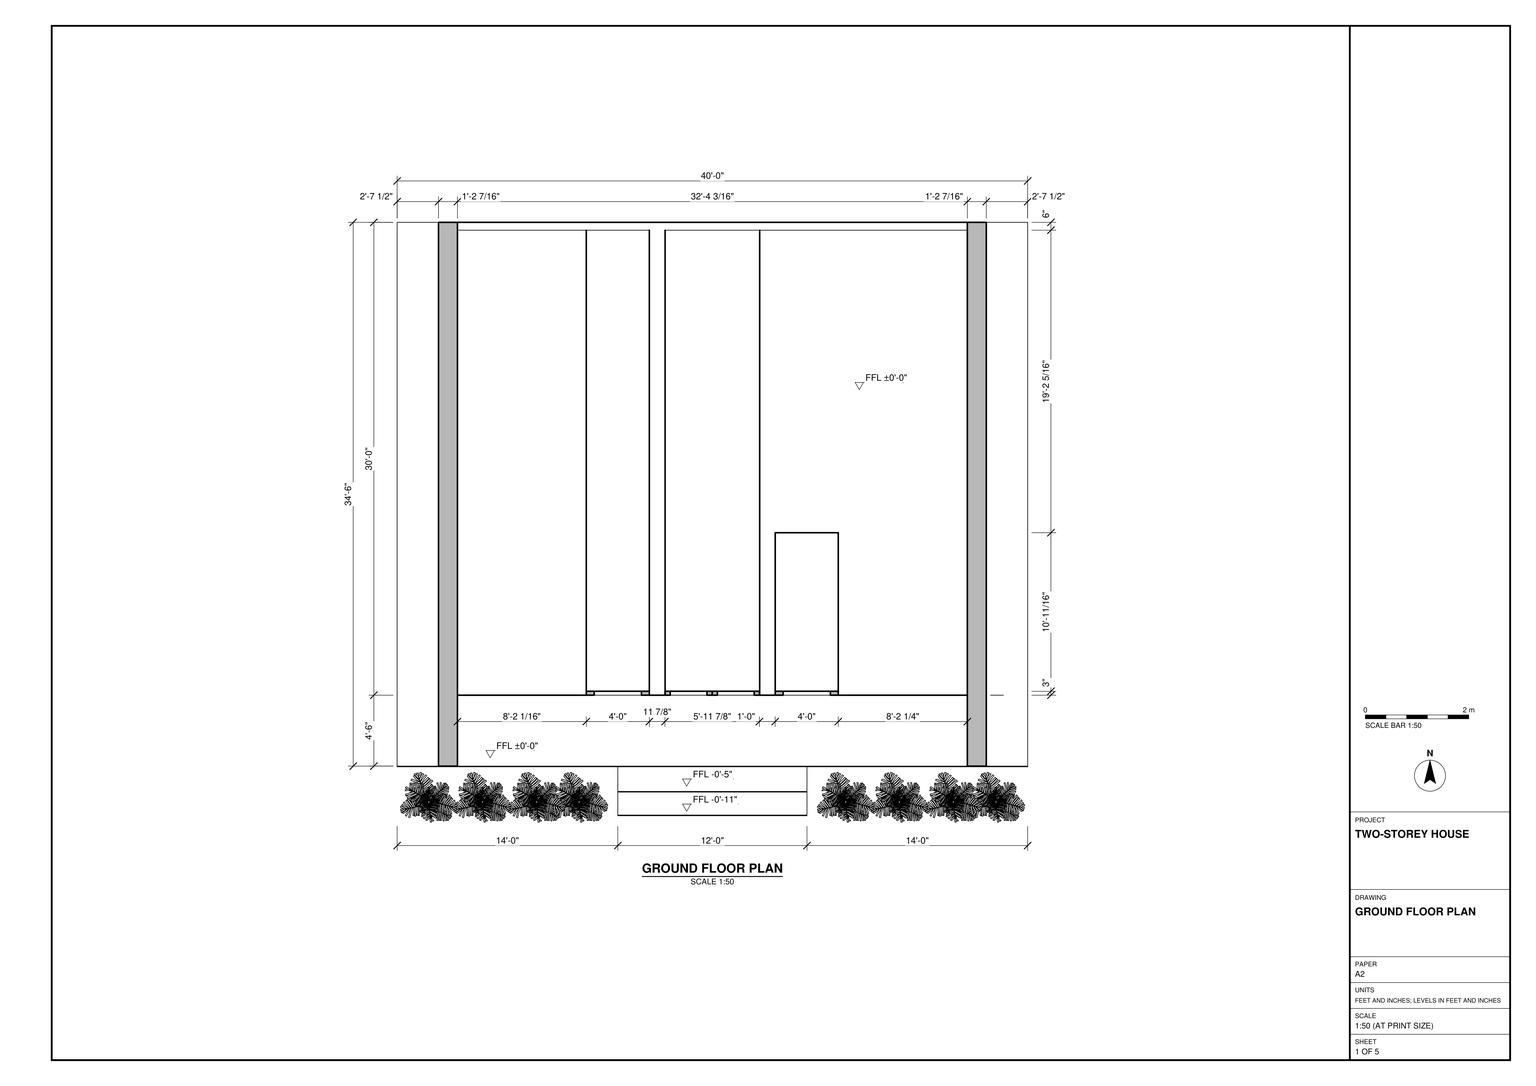
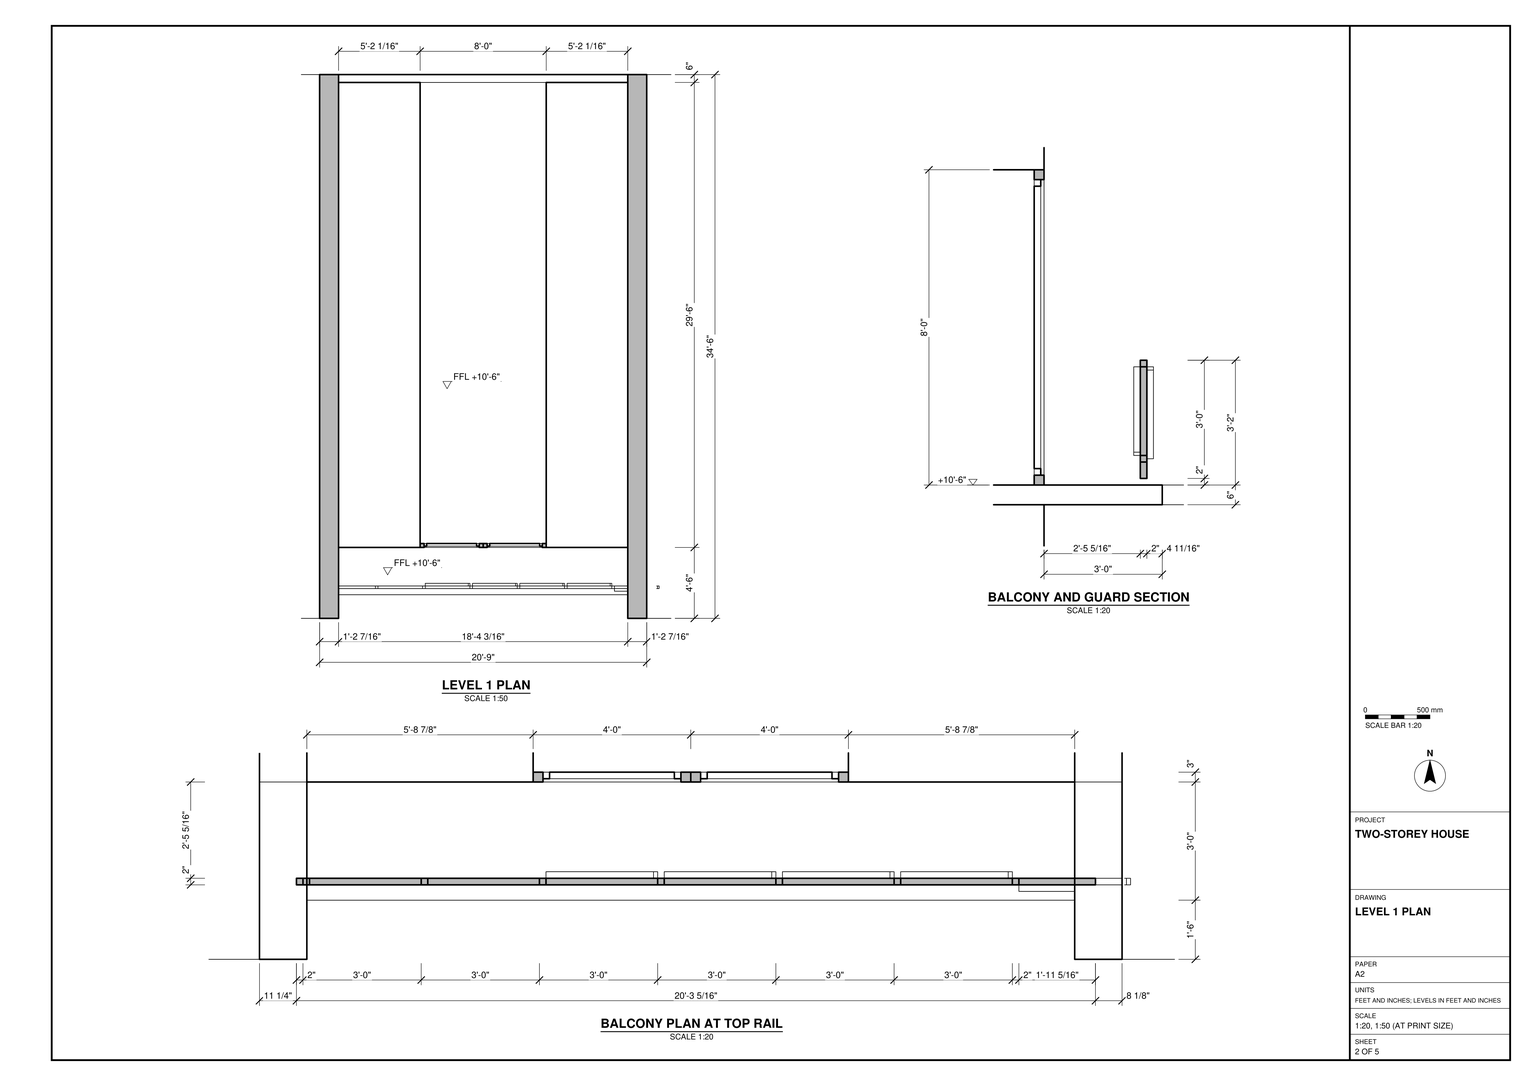
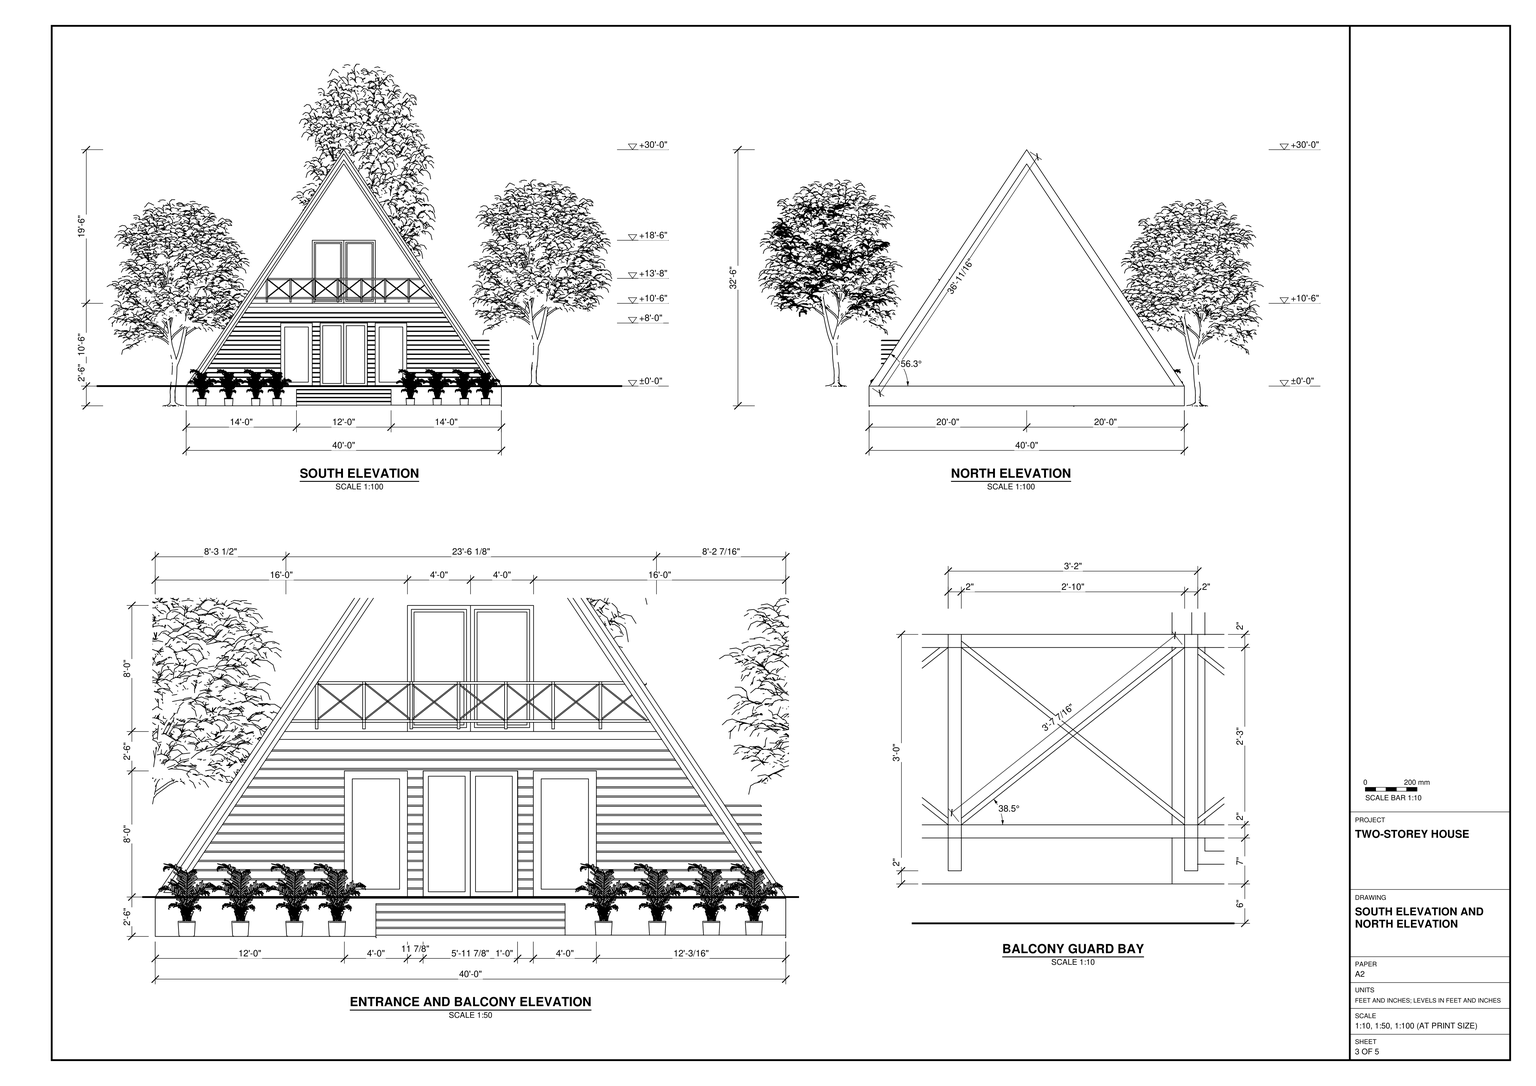
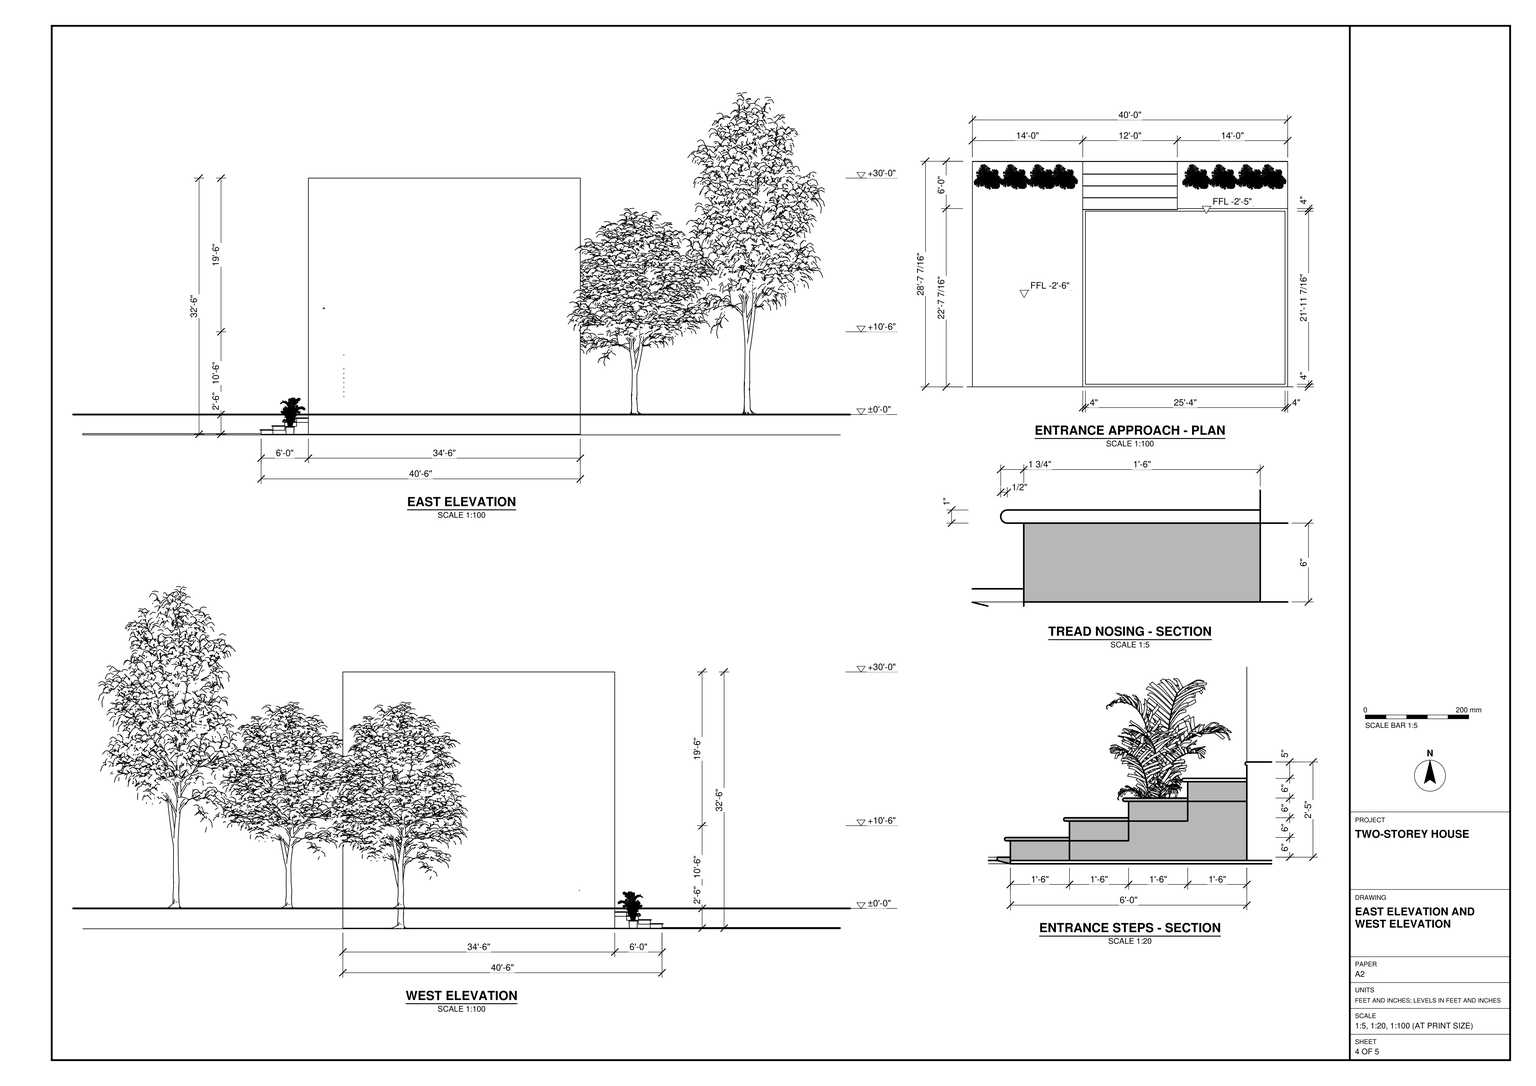
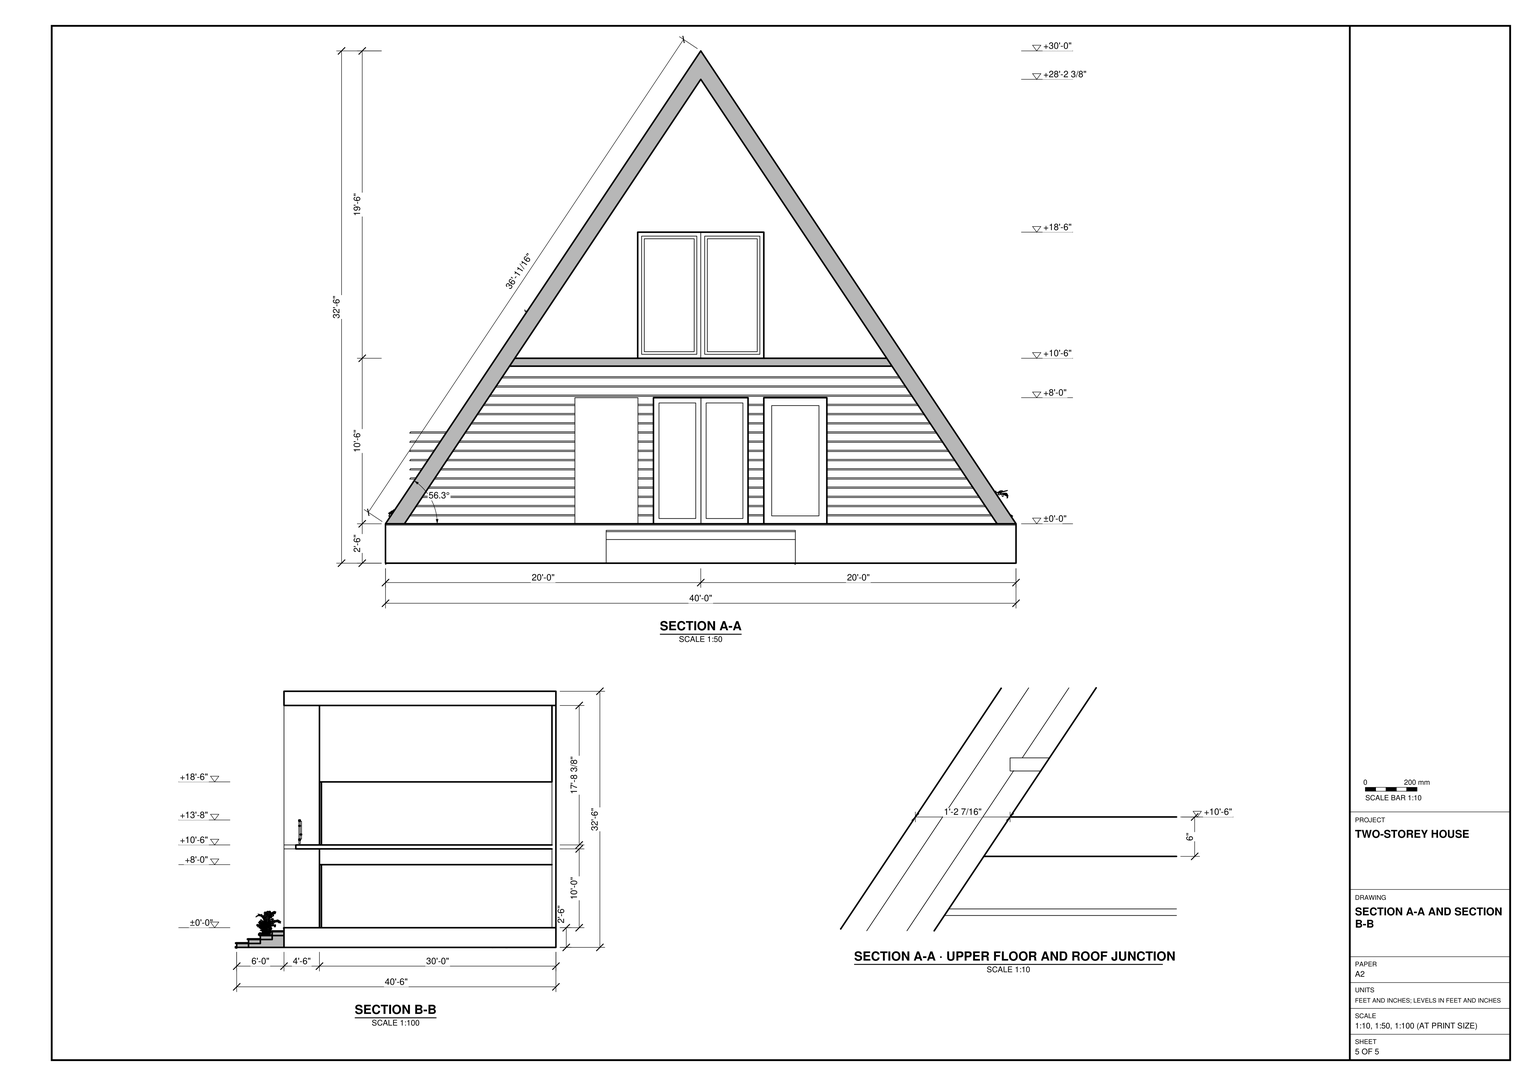
Build the A-frame house and its setting in SketchUp from task_files/diagram_01.pdf. Work in feet and inches. The complete model, including the site elements, measures 147'-9/16" along X, 111'-6 13/16" along Y and 43'-5 1/4" along Z. Set the ground floor at ±0'-0" and the upper floor at +10'-6".

Make the house base 40'-0" across the gable and 34'-6" from front to back, excluding the entrance steps. Run the ridge from south to north, with both roof slopes descending to the sides of the base. Follow the plans for the wall positions and thicknesses. Recess the south entrance beneath the roof, model the horizontal courses around its framed openings, and centre the entrance steps between the rows of plants.

Fit the narrower upper floor between the roof slopes. Place the paired upper doors behind the projecting balcony slab. Use the balcony plan, section and guard detail to position the posts, rails and crossed diagonals. Include the surrounding trees as shown. Decor and loose items, including plants, may be any suitable library components.

Keep the walls, slabs, roof and steps separately grouped, and make each furniture or joinery piece shown a separate group or component. Use components for repeated parts such as guard bays. Save one SketchUp model as output_files/two_storey_a_frame_house_with_a_front_balcony.skp.

# SketchUp Ruby script. Lengths in inches.
U = 1.inch
M = Sketchup.active_model
def pt(a) = Geom::Point3d.new(a.map { |v| v * U })
def face(e, loops, mat)
  f = e.add_face(loops[0].map { |a| pt(a) })
  loops[1..].each { |l| e.add_face(l.map { |a| pt(a) }).erase! }
  f.material = f.back_material = mat if mat
  f
end
# faces: each face lists its corners as indices into pts; further lists are holes
def faces(e, pts, list, mat = nil) = list.each { |f| face(e, (f[0].is_a?(Array) ? f : [f]).map { |l| l.map { |i| pts[i] } }, mat) }
# xy, xz, yz: faces in a plane at the given z, y or x. An outline is a flat list of corners, or four numbers for a rectangle; further outlines are holes
def ring(l) = l.size == 4 ? [[l[0], l[1]], [l[2], l[1]], [l[2], l[3]], [l[0], l[3]]] : l.each_slice(2).to_a
def flat(e, list, mat, &to3) = list.each { |f| face(e, (f[0].is_a?(Array) ? f : [f]).map { |l| ring(l).map { |u, v| to3.(u, v) } }, mat) }
def xy(e, z, list, mat = nil) = flat(e, list, mat) { |x, y| [x, y, z] }
def xz(e, y, list, mat = nil) = flat(e, list, mat) { |x, z| [x, y, z] }
def yz(e, x, list, mat = nil) = flat(e, list, mat) { |y, z| [x, y, z] }
def lines(e, pts, list) = list.each { |a, b| e.add_line(pt(pts[a]), pt(pts[b])) }
# prism: a flat outline (further loops are holes) pulled along v
def prism(e, loops, v, mat = nil)
  f = face(e, loops, mat); d = Geom::Vector3d.new(v.map { |x| x * U })
  f.pushpull(f.normal.samedirection?(d) ? d.length : -d.length)
end
def box(e, o, s, mat = nil) = prism(e, [[o, [o[0] + s[0], o[1], o[2]], [o[0] + s[0], o[1] + s[1], o[2]], [o[0], o[1] + s[1], o[2]]]], [0, 0, s[2]], mat)
def at(x, y, z, deg = 0) = Geom::Transformation.translation(pt([x, y, z])) * Geom::Transformation.rotation(ORIGIN, Z_AXIS, deg.degrees)
def axes(o, x, y, z) = Geom::Transformation.new([*x, 0, *y, 0, *z, 0, *pt(o).to_a, 1])
def part(name) = M.definitions.add(name)
# library, detail: a bought-in or finely detailed component or shape, given as its bounding box
def library(name, o, s) = part(name).tap { |d| box(d.entities, o, s) }
def detail(e, o, s) = box(e.add_group.entities, o, s)
def put(e, d, t, mat = nil) = e.add_instance(d, t).tap { |i| i.material = mat if mat }
def group(e, t, mat = nil) = e.add_group.tap { |g| g.transformation = t; g.material = mat if mat }.entities
root = M.entities
M.materials.add("AM171_024").color = [90, 82, 72]
M.materials.add("AM171_1").color = [185, 198, 172]
M.materials.add("[Brick Colored Blue]").color = [144, 143, 146]
M.materials.add("[Color M07]").color = [58, 58, 58]
M.materials.add("[Grass Dark Green]").color = [106, 157, 55]
M.materials.add("[Groundcover Bark Chips]").color = [119, 116, 116]
M.materials.add("[Translucent Glass Gray]").color = [128, 128, 128]
M.materials["[Translucent Glass Gray]"].alpha = 0.5
M.materials.add("[Wood Cherry Original]").color = [152, 86, 42]
c1 = library("AM171_024_Defintion",[-287.72,-290.04,-2.17],[634.47,642.61,1000])
c2 = library("AM171_024_Defintion1",[-419.22,-426.02,309.0625],[911.71,919.28,1000])
c3 = part("SG-+Cay+Via+he")
g1 = group(c3.entities,at(0,0,0))
put(g1,c1,axes([0,0,0],[0.30662,0,0],[0,0.30662,0],[0,0,0.30662]),"AM171_024")
put(g1,c2,axes([0,0,0],[0.23988,0,0],[0,0.23988,0],[0,0,0.23988]),"AM171_1")
c4 = part("Group\#6")
xy(c4.entities,0,[[0,0,48,3]],"[Color M07]")
xy(c4.entities,6,[[6,0,42,3]],"[Color M07]")
xy(c4.entities,90,[[6,0,42,3]],"[Color M07]")
xy(c4.entities,96,[[0,0,48,3]],"[Color M07]")
xz(c4.entities,0,[[[0,0,48,96],[6,6,42,90]]],"[Color M07]")
xz(c4.entities,3,[[[0,0,48,96],[6,6,42,90]]])
xz(c4.entities,3,[[6,6,42,90]],"[Translucent Glass Gray]")
yz(c4.entities,0,[[0,0,3,96]],"[Color M07]")
yz(c4.entities,6,[[0,6,3,90]],"[Color M07]")
yz(c4.entities,42,[[0,6,3,90]],"[Color M07]")
yz(c4.entities,48,[[0,0,3,96]],"[Color M07]")
c5 = part("Group\#7")
xy(c5.entities,0,[[0,0,36,3]],"[Color M07]")
xy(c5.entities,4,[[4,0,32,3]],"[Color M07]")
xy(c5.entities,92,[[4,0,32,3]],"[Color M07]")
xy(c5.entities,96,[[0,0,36,3]],"[Color M07]")
xz(c5.entities,0,[[[0,0,36,96],[4,4,32,92]]],"[Color M07]")
xz(c5.entities,3,[[[0,0,36,96],[4,4,32,92]]],"[Color M07]")
xz(c5.entities,3,[[4,4,32,92]],"[Translucent Glass Gray]")
yz(c5.entities,0,[[0,0,3,96]],"[Color M07]")
yz(c5.entities,4,[[0,4,3,92]],"[Color M07]")
yz(c5.entities,32,[[0,4,3,92]],"[Color M07]")
yz(c5.entities,36,[[0,0,3,96]],"[Color M07]")
c6 = part("Group\#8")
box(c6.entities,[0,18,0],[144,18,6])
c7 = part("Group\#5")
prism(c7.entities,[[[144,-1.26,0],[144,18,0],[144,18,1],[144,-1.26,1],[144,-1.39,0.98],[144,-1.51,0.93],[144,-1.61,0.85],[144,-1.69,0.75],[144,-1.74,0.63],[144,-1.76,0.5],[144,-1.74,0.37],[144,-1.69,0.25],[144,-1.61,0.15],[144,-1.51,0.07],[144,-1.39,0.02]]],[-144,0,0])
c8 = part("Group\#9")
xy(c8.entities,0,[[0,0,48,3]],"[Color M07]")
xy(c8.entities,3,[[3,1,45,3]])
xy(c8.entities,3,[[3,0,45,1]],"[Color M07]")
xy(c8.entities,5,[[5,1,43,3]])
xy(c8.entities,91,[[5,1,43,3]])
xy(c8.entities,93,[[3,1,45,3]])
xy(c8.entities,93,[[3,0,45,1]],"[Color M07]")
xy(c8.entities,96,[[0,0,48,3]],"[Color M07]")
xz(c8.entities,0,[[[0,0,48,96],[3,3,45,93]]],"[Color M07]")
xz(c8.entities,1,[[[3,3,45,93],[5,5,43,91]]],"[Color M07]")
xz(c8.entities,3,[[[0,0,48,96],[3,3,45,93]]])
xz(c8.entities,3,[[5,5,43,91]],"[Translucent Glass Gray]")
yz(c8.entities,0,[[0,0,3,96]],"[Color M07]")
yz(c8.entities,3,[[1,3,3,93]])
yz(c8.entities,3,[[0,3,1,93]],"[Color M07]")
yz(c8.entities,5,[[1,5,3,91]])
yz(c8.entities,43,[[1,5,3,91]])
yz(c8.entities,45,[[1,3,3,93]])
yz(c8.entities,45,[[0,3,1,93]],"[Color M07]")
yz(c8.entities,48,[[0,0,3,96]])
c9 = part("Group\#14")
prism(c9.entities,[[[0,0,28],[0,0,27],[34,0,0],[34,0,1]]],[0,2,0])
c10 = part("Group\#12")
box(c10.entities,[0,0,0],[2,2,36])
c11 = part("Group\#15")
prism(c11.entities,[[[0,2,1],[32.74,2,27],[34,2,27],[0,2,0]]],[0,-2,0])
p = [[34,0,28],[34,0,27]]
lines(c11.entities,p,[[0,1]])
c12 = library("Group\#22",[-1.74,-3.05,0],[161.91,43.96,59.125])
put(root,c3,at(297.05,669.42,-30))
put(root,c3,at(847,839.78,0))
put(root,c3,at(59.55,669.42,0))
put(root,c3,axes([578.13,1011.46,0.37],[1,0,0],[0,1,0],[0,0,1.56]))
g2 = group(root,at(317,397.4375,0),"[Wood Cherry Original]")
xy(g2,0,[[0,-54,14.42,360],[465.58,-54,480,360],[14.42,0,144,354],[192,0,192,354,14.42,354,14.42,360,465.58,360,465.58,354,204,354,204,0],[276,0,276,354,465.58,354,465.58,0,335.8125,0,335.8125,123.6875,287.8125,123.6875,287.8125,0]])
xy(g2,96,[[144,0,192,354],[204,0,276,354],[287.8125,0,335.8125,123.6875]])
xy(g2,120,[[94.42,-36,385.58,0],[94.42,0,385.58,354]])
xy(g2,126,[[98.42,-36,381.58,-36,381.58,0,288,0,288,354,192,354,192,0,98.42,0],[98.42,0,192,354],[288,0,381.58,354]])
xy(g2,222,[[192,0,288,354]])
xz(g2,-54,[[[0,0,14.42,0,240,338.37,465.58,0,480,0,240,360],[6.45,3.45,240,353.77,473.55,3.45,467.43,3.45,384.45,127.92,240,344.59,95.55,127.92,12.57,3.45]],[6.45,3.45,12.57,3.45,95.55,127.92,240,344.59,384.45,127.92,467.43,3.45,473.55,3.45,240,353.77]],"[Color M07]")
xz(g2,-36,[[94.42,120,385.58,120,381.58,126,98.42,126]],"[Color M07]")
xz(g2,0,[[14.42,0,144,0,144,6,18.42,6],[192,0,204,6],[276,0,287.8125,6],[335.8125,0,465.58,0,461.58,6,335.8125,6],[18.42,6,144,6,144,7,19.09,7],
  [192,6,204,7],[276,6,287.8125,7],[335.8125,6,461.58,6,460.91,7,335.8125,7],[19.09,7,144,7,144,13,23.09,13],[192,7,204,13],
  [276,7,287.8125,13],[335.8125,7,460.91,7,456.91,13,335.8125,13],[18.42,13,23.09,13,23.76,14,19.09,14],[23.09,13,144,13,144,14,23.76,14],[192,13,204,14],
  [276,13,287.8125,14],[335.8125,13,456.91,13,456.24,14,335.8125,14],[456.91,13,461.58,13,460.91,14,456.24,14],[23.76,14,144,14,144,20,27.76,20],[192,14,204,20],
  [276,14,287.8125,20],[335.8125,14,456.24,14,452.24,20,335.8125,20],[18.42,20,27.76,20,28.42,21,19.09,21],[27.76,20,144,20,144,21,28.42,21],[192,20,204,21],
  [276,20,287.8125,21],[335.8125,20,452.24,20,451.58,21,335.8125,21],[452.24,20,461.58,20,460.91,21,451.58,21],[28.42,21,144,21,144,27,32.42,27],[192,21,204,27],
  [276,21,287.8125,27],[335.8125,21,451.58,21,447.58,27,335.8125,27],[18.42,27,32.42,27,33.09,28,19.09,28],[32.42,27,144,27,144,28,33.09,28],[192,27,204,28],
  [276,27,287.8125,28],[335.8125,27,447.58,27,446.91,28,335.8125,28],[447.58,27,461.58,27,460.91,28,446.91,28],[33.09,28,144,28,144,34,37.09,34],[192,28,204,34],
  [276,28,287.8125,34],[335.8125,28,446.91,28,442.91,34,335.8125,34],[37.09,34,144,34,144,35,37.76,35],[192,34,204,35],[276,34,287.8125,35],
  [335.8125,34,442.91,34,442.24,35,335.8125,35],[442.91,34,461.58,34,460.91,35,442.24,35],[37.76,35,144,35,144,41,41.76,41],[192,35,204,41],[276,35,287.8125,41],
  [335.8125,35,442.24,35,438.24,41,335.8125,41],[41.76,41,144,41,144,42,42.42,42],[192,41,204,42],[276,41,287.8125,42],[335.8125,41,438.24,41,437.58,42,335.8125,42],
  [438.24,41,461.58,41,460.91,42,437.58,42],[42.42,42,144,42,144,48,46.42,48],[192,42,204,48],[276,42,287.8125,48],[335.8125,42,437.58,42,433.58,48,335.8125,48],
  [46.42,48,144,48,144,49,47.09,49],[192,48,204,49],[276,48,287.8125,49],[335.8125,48,433.58,48,432.91,49,335.8125,49],[433.58,48,461.58,48,460.91,49,432.91,49],
  [47.09,49,144,49,144,55,51.09,55],[192,49,204,55],[276,49,287.8125,55],[335.8125,49,432.91,49,428.91,55,335.8125,55],[51.09,55,144,55,144,56,51.76,56],
  [192,55,204,56],[276,55,287.8125,56],[335.8125,55,428.91,55,428.24,56,335.8125,56],[428.91,55,461.58,55,460.91,56,428.24,56],[51.76,56,144,56,144,62,55.76,62],
  [192,56,204,62],[276,56,287.8125,62],[335.8125,56,428.24,56,424.24,62,335.8125,62],[55.76,62,144,62,144,63,56.42,63],[192,62,204,63],
  [276,62,287.8125,63],[335.8125,62,424.24,62,423.58,63,335.8125,63],[424.24,62,461.58,62,460.91,63,423.58,63],[56.42,63,144,63,144,69,60.42,69],[192,63,204,69],
  [276,63,287.8125,69],[335.8125,63,423.58,63,419.58,69,335.8125,69],[60.42,69,144,69,144,70,61.09,70],[192,69,204,70],[276,69,287.8125,70],
  [335.8125,69,419.58,69,418.91,70,335.8125,70],[419.58,69,461.58,69,460.91,70,418.91,70],[61.09,70,144,70,144,76,65.09,76],[192,70,204,76],[276,70,287.8125,76],
  [335.8125,70,418.91,70,414.91,76,335.8125,76],[65.09,76,144,76,144,77,65.76,77],[192,76,204,77],[276,76,287.8125,77],[335.8125,76,414.91,76,414.24,77,335.8125,77],
  [414.91,76,419.58,76,418.91,77,414.24,77],[65.76,77,144,77,144,83,69.76,83],[192,77,204,83],[276,77,287.8125,83],[335.8125,77,414.24,77,410.24,83,335.8125,83],
  [69.76,83,144,83,144,84,70.42,84],[192,83,204,84],[276,83,287.8125,84],[335.8125,83,410.24,83,409.58,84,335.8125,84],[410.24,83,419.58,83,418.91,84,409.58,84],
  [70.42,84,144,84,144,90,74.42,90],[192,84,204,90],[276,84,287.8125,90],[335.8125,84,409.58,84,405.58,90,335.8125,90],[74.42,90,144,90,144,91,75.09,91],
  [192,90,204,91],[276,90,287.8125,91],[335.8125,90,405.58,90,404.91,91,335.8125,91],[405.58,90,419.58,90,418.91,91,404.91,91],[75.09,91,144,91,144,96,192,96,192,91,204,91,204,96,276,96,276,91,287.8125,91,287.8125,96,335.8125,96,335.8125,91,404.91,91,400.91,97,79.09,97],
  [79.09,97,400.91,97,400.24,98,79.76,98],[79.76,98,400.24,98,396.24,104,83.76,104],[83.76,104,396.24,104,395.58,105,84.42,105],[84.42,105,395.58,105,391.58,111,88.42,111],[88.42,111,391.58,111,390.91,112,89.09,112],
  [89.09,112,390.91,112,385.58,120,94.42,120],[98.42,126,192,126,192,222,288,222,288,126,381.58,126,240,338.37]])
xz(g2,123.6875,[[287.8125,0,335.8125,96]])
xz(g2,354,[[98.42,126,192,126,192,222,288,222,288,126,381.58,126,240,338.37]])
xz(g2,360,[[0,0,240,360,480,0,465.58,0,240,338.37,14.42,0],[14.42,0,240,338.37,465.58,0]])
yz(g2,144,[[0,0,354,96]])
yz(g2,192,[[0,0,354,96],[0,126,354,222]])
yz(g2,204,[[0,0,354,96]])
yz(g2,276,[[0,0,354,96]])
yz(g2,287.8125,[[0,0,123.6875,96]])
yz(g2,288,[[0,126,354,222]])
yz(g2,335.8125,[[0,0,123.6875,96]])
p = [[0,360,0],[0,-54,0],[240,-54,360],[240,360,360],[89.09,0,112],[94.42,0,120],
  [94.42,-36,120],[94.42,-54,120],[14.42,-54,0],[14.42,0,0],[18.42,0,6],[19.09,0,7],
  [23.09,0,13],[23.76,0,14],[27.76,0,20],[28.42,0,21],[32.42,0,27],[33.09,0,28],
  [37.09,0,34],[37.76,0,35],[41.76,0,41],[42.42,0,42],[46.42,0,48],[47.09,0,49],
  [51.09,0,55],[51.76,0,56],[55.76,0,62],[56.42,0,63],[60.42,0,69],[61.09,0,70],
  [65.09,0,76],[65.76,0,77],[69.76,0,83],[70.42,0,84],[74.42,0,90],[75.09,0,91],
  [79.09,0,97],[79.76,0,98],[83.76,0,104],[84.42,0,105],[88.42,0,111],[480,-54,0],
  [480,360,0],[465.58,0,0],[465.58,-54,0],[385.58,-54,120],[385.58,-36,120],[385.58,0,120],
  [390.91,0,112],[391.58,0,111],[395.58,0,105],[396.24,0,104],[400.24,0,98],[400.91,0,97],
  [404.91,0,91],[405.58,0,90],[409.58,0,84],[410.24,0,83],[414.24,0,77],[414.91,0,76],
  [418.91,0,70],[419.58,0,69],[423.58,0,63],[424.24,0,62],[428.24,0,56],[428.91,0,55],
  [432.91,0,49],[433.58,0,48],[437.58,0,42],[438.24,0,41],[442.24,0,35],[442.91,0,34],
  [446.91,0,28],[447.58,0,27],[451.58,0,21],[452.24,0,20],[456.24,0,14],[456.91,0,13],
  [460.91,0,7],[461.58,0,6],[14.42,360,0],[240,360,338.37],[240,354,338.37],[98.42,354,126],
  [98.42,0,126],[98.42,-36,126],[94.42,354,120],[14.42,354,0],[465.58,360,0],[465.58,354,0],
  [385.58,354,120],[381.58,-36,126],[381.58,0,126],[381.58,354,126],[98.42,-54,126],[381.58,-54,126],
  [240,0,338.37],[240,-54,338.37],[14.42,0,6],[18.42,0,7],[14.42,0,7],[465.58,0,6],
  [461.58,0,7]]
faces(g2,p,[[0,1,2,3],[3,2,41,42],[6,85,94,7],[91,46,45,95]],"[Color M07]")
faces(g2,p,[[4,5,6,7,8,9,10,11,12,13,14,15,16,17,18,19,20,21,22,23,24,25,26,27,28,29,30,31,32,33,34,35,36,37,38,39,40],[43,44,45,46,47,48,49,50,51,52,53,54,55,56,57,58,59,60,61,62,63,64,65,66,67,68,69,70,71,72,73,74,75,76,77,78,79],[80,81,82,83,84,85,6,5,86,87],[81,88,89,90,47,46,91,92,93,82],[86,5,4,40,39,38,37,36,35,34,33,32,31,30,29,28,27,26,25,24,23,22,21,20,19,18,17,16,15,14,13,12,11,10,9,87],[43,79,78,77,76,75,74,73,72,71,70,69,68,67,66,65,64,63,62,61,60,59,58,57,56,55,54,53,52,51,50,49,48,47,90,89],[96,97,94,85,84],[97,96,92,91,95],
  [82,96,84,83],[93,92,96,82]])
lines(g2,p,[[98,10],[99,11],[100,99],[79,101],[78,102]])
put(g2,c4,at(144,0,0))
put(g2,c5,at(203.91,0,0))
put(g2,c5,at(239.8125,0,0))
put(g2,c4,at(287.8125,0,0))
g3 = group(root,at(317,361.4375,-48))
xy(g3,18,[[0,-18,480,396]])
xy(g3,48,[[0,-18,480,396]],"[Brick Colored Blue]")
xz(g3,-18,[[0,18,480,47]],"[Brick Colored Blue]")
xz(g3,396,[[0,18,480,48]])
yz(g3,0,[[-18,18,-18,47,-18.13,47.02,-18.25,47.07,-18.35,47.15,-18.43,47.25,-18.48,47.37,-18.5,47.5,-18.48,47.63,-18.43,47.75,-18.35,47.85,-18.25,47.93,-18.13,47.98,-18,48,396,48,396,18]],"[Brick Colored Blue]")
yz(g3,480,[[-18,18,396,18,396,48,-18,48,-18.13,47.98,-18.25,47.93,-18.35,47.85,-18.43,47.75,-18.48,47.63,-18.5,47.5,-18.48,47.37,-18.43,47.25,-18.35,47.15,-18.25,47.07,-18.13,47.02,-18,47]],"[Brick Colored Blue]")
p = [[0,-18.25,47.07],[0,-18.13,47.02],[480,-18.13,47.02],[480,-18.25,47.07],[0,-18,47],[480,-18,47],
  [0,-18.43,47.25],[0,-18.35,47.15],[480,-18.35,47.15],[480,-18.43,47.25],[0,-18.48,47.37],[480,-18.48,47.37],
  [0,-18.5,47.5],[480,-18.5,47.5],[0,-18.48,47.63],[480,-18.48,47.63],[0,-18.43,47.75],[480,-18.43,47.75],
  [0,-18.35,47.85],[480,-18.35,47.85],[0,-18.25,47.93],[480,-18.25,47.93],[0,-18.13,47.98],[480,-18.13,47.98],
  [0,-18,48],[480,-18,48]]
faces(g3,p,[[0,1,2,3],[1,4,5,2],[6,7,8,9],[7,0,3,8],[10,6,9,11],[12,10,11,13],[14,12,13,15],[16,14,15,17],
  [18,16,17,19],[20,18,19,21],[22,20,21,23],[24,22,23,25]])
put(root,c6,at(485,307.4375,-12),"[Brick Colored Blue]")
put(root,c6,at(485,289.4375,-18),"[Brick Colored Blue]")
g4 = group(root,at(485,271.4375,-24),"[Brick Colored Blue]")
box(g4,[0,18,0],[144,18,6])
put(root,c6,at(485,253.4375,-30),"[Brick Colored Blue]")
g5 = group(root,at(485,289.4375,-30),"[Brick Colored Blue]")
prism(g5,[[[144,0,6],[144,0,0],[144,54,0],[144,54,18],[144,36,18],[144,36,12],[144,18,12],[144,18,6]]],[-144,0,0])
put(root,c7,at(485,325.4375,-6))
put(root,c7,at(485,307.4375,-12))
put(root,c7,at(485,289.4375,-18))
put(root,c7,at(485,271.4375,-24))
put(root,c8,at(509,397.4375,126))
put(root,c8,at(557,397.4375,126),"[Color M07]")
put(root,c9,at(440.91,366.12,135),"[Color M07]")
g6 = group(root,at(416.48,366.12,126),"[Color M07]")
g7 = group(g6,at(0,0,7))
prism(g7,[[[0,0,0],[282.1,0,0],[282.1,0,2],[18,0,2],[0,0,2]]],[0,2,0])
put(g6,c10,at(22.4375,0,2))
put(g6,c10,at(58.4375,0,2))
put(g6,c10,at(94.4375,0,2))
put(g6,c10,at(130.4375,0,2))
put(g6,c10,at(166.4375,0,2))
put(g6,c10,at(202.4375,0,2))
put(g6,c10,at(238.4375,0,2))
g8 = group(g6,at(0,0,36))
xy(g8,0,[[20.45,0,263.75,2]])
xy(g8,2,[[18,0,20.45,2],[20.45,0,263.75,2]])
xz(g8,0,[[20.45,0,263.75,2]])
xz(g8,2,[[20.45,0,263.75,2]])
yz(g8,20.45,[[0,0,2,2]])
yz(g8,263.75,[[0,0,2,2]])
put(root,c11,at(440.91,366.12,135),"[Color M07]")
put(root,c9,at(476.91,366.12,135),"[Color M07]")
put(root,c11,at(476.91,366.12,135),"[Color M07]")
put(root,c9,at(512.91,366.12,134),"[Color M07]")
put(root,c11,at(512.91,368.12,135),"[Color M07]")
put(root,c9,at(548.91,366.12,134),"[Color M07]")
put(root,c11,at(548.91,368.12,135),"[Color M07]")
put(root,c11,at(584.91,368.12,135),"[Color M07]")
put(root,c9,at(584.91,366.12,134),"[Color M07]")
put(root,c11,at(620.91,368.12,135),"[Color M07]")
put(root,c9,at(620.91,366.12,134),"[Color M07]")
put(root,c11,at(656.91,366.12,135),"[Color M07]")
put(root,c9,at(656.91,364.12,134),"[Color M07]")
g9 = group(root,at(317,271.4375,-30),"[Grass Dark Green]")
xy(g9,0,[[0,-271.4375,168,72]])
g10 = group(root,at(629,271.4375,-30),"[Grass Dark Green]")
xy(g10,0,[[0,0,168,72]])
put(root,c12,at(636.83,300.68,-30))
put(root,c12,at(319.45,300.68,-30))
g11 = group(root,at(0,0,-31))
xy(g11,0,[[0,0,0,1338.8125,1723.5625,1338.8125,1723.5625,0,797,0,797,271.4375,485,271.4375,485,0]],"[Grass Dark Green]")
xy(g11,1,[[489,4,793,267.4375]],"[Groundcover Bark Chips]")
xy(g11,2,[[[485,0,797,271.4375],[489,4,793,267.4375]]],"[Groundcover Bark Chips]")
xz(g11,0,[[485,0,797,2]],"[Groundcover Bark Chips]")
xz(g11,4,[[489,1,793,2]],"[Groundcover Bark Chips]")
xz(g11,267.4375,[[489,1,793,2]],"[Groundcover Bark Chips]")
xz(g11,271.4375,[[485,0,797,2]],"[Groundcover Bark Chips]")
yz(g11,485,[[0,0,271.4375,2]],"[Groundcover Bark Chips]")
yz(g11,489,[[4,1,267.4375,2]],"[Groundcover Bark Chips]")
yz(g11,793,[[4,1,267.4375,2]],"[Groundcover Bark Chips]")
yz(g11,797,[[0,0,271.4375,2]],"[Groundcover Bark Chips]")
p = [[485,0,0],[485,271.4375,0],[489,267.4375,1],[489,4,1],[797,0,0],[793,4,1],
  [797,271.4375,0],[793,267.4375,1]]
faces(g11,p,[[0,1,2,3],[4,0,3,5],[6,4,5,7],[1,6,7,2]],"[Groundcover Bark Chips]")
